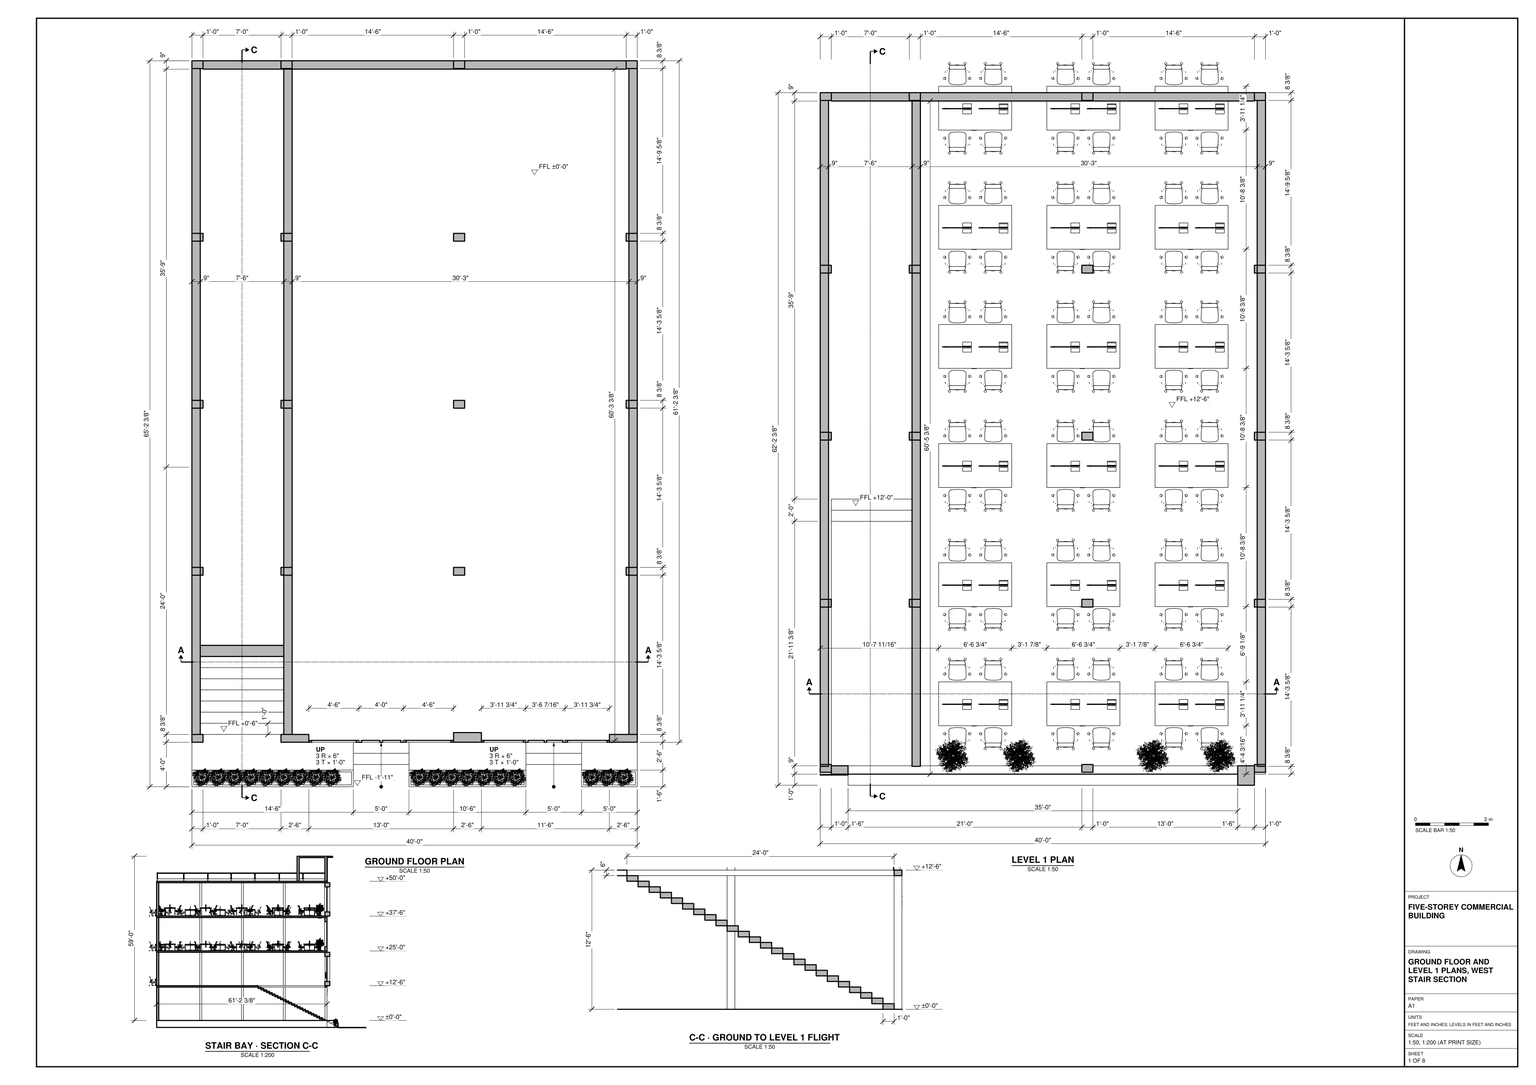
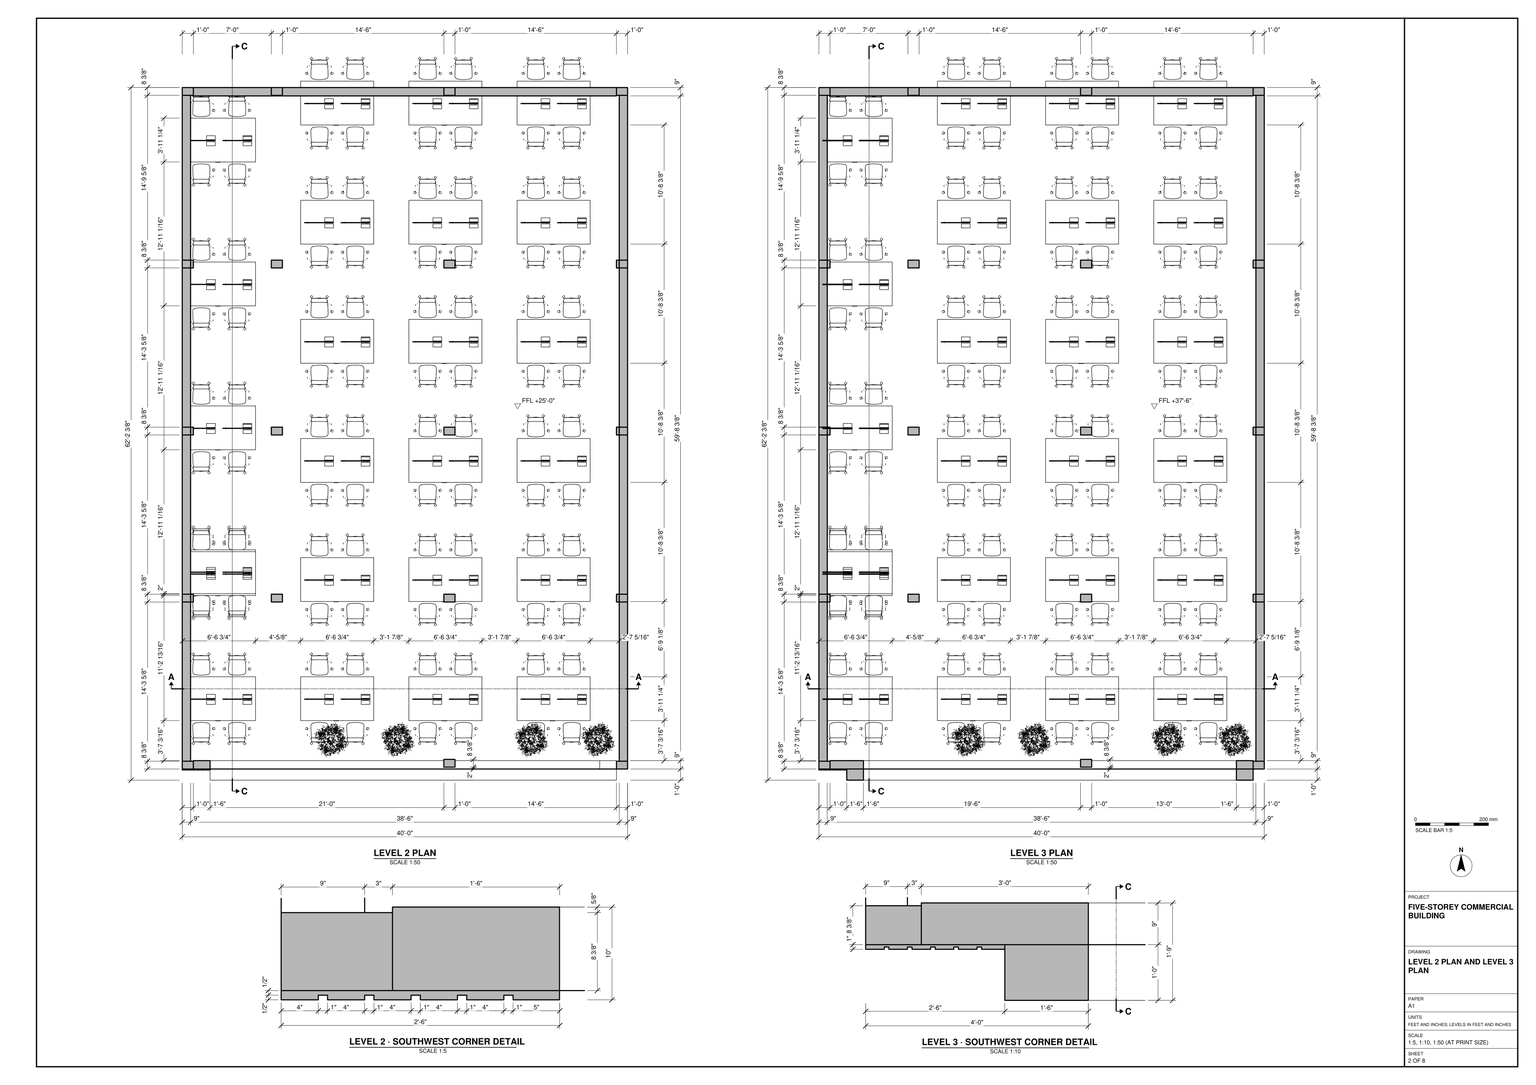
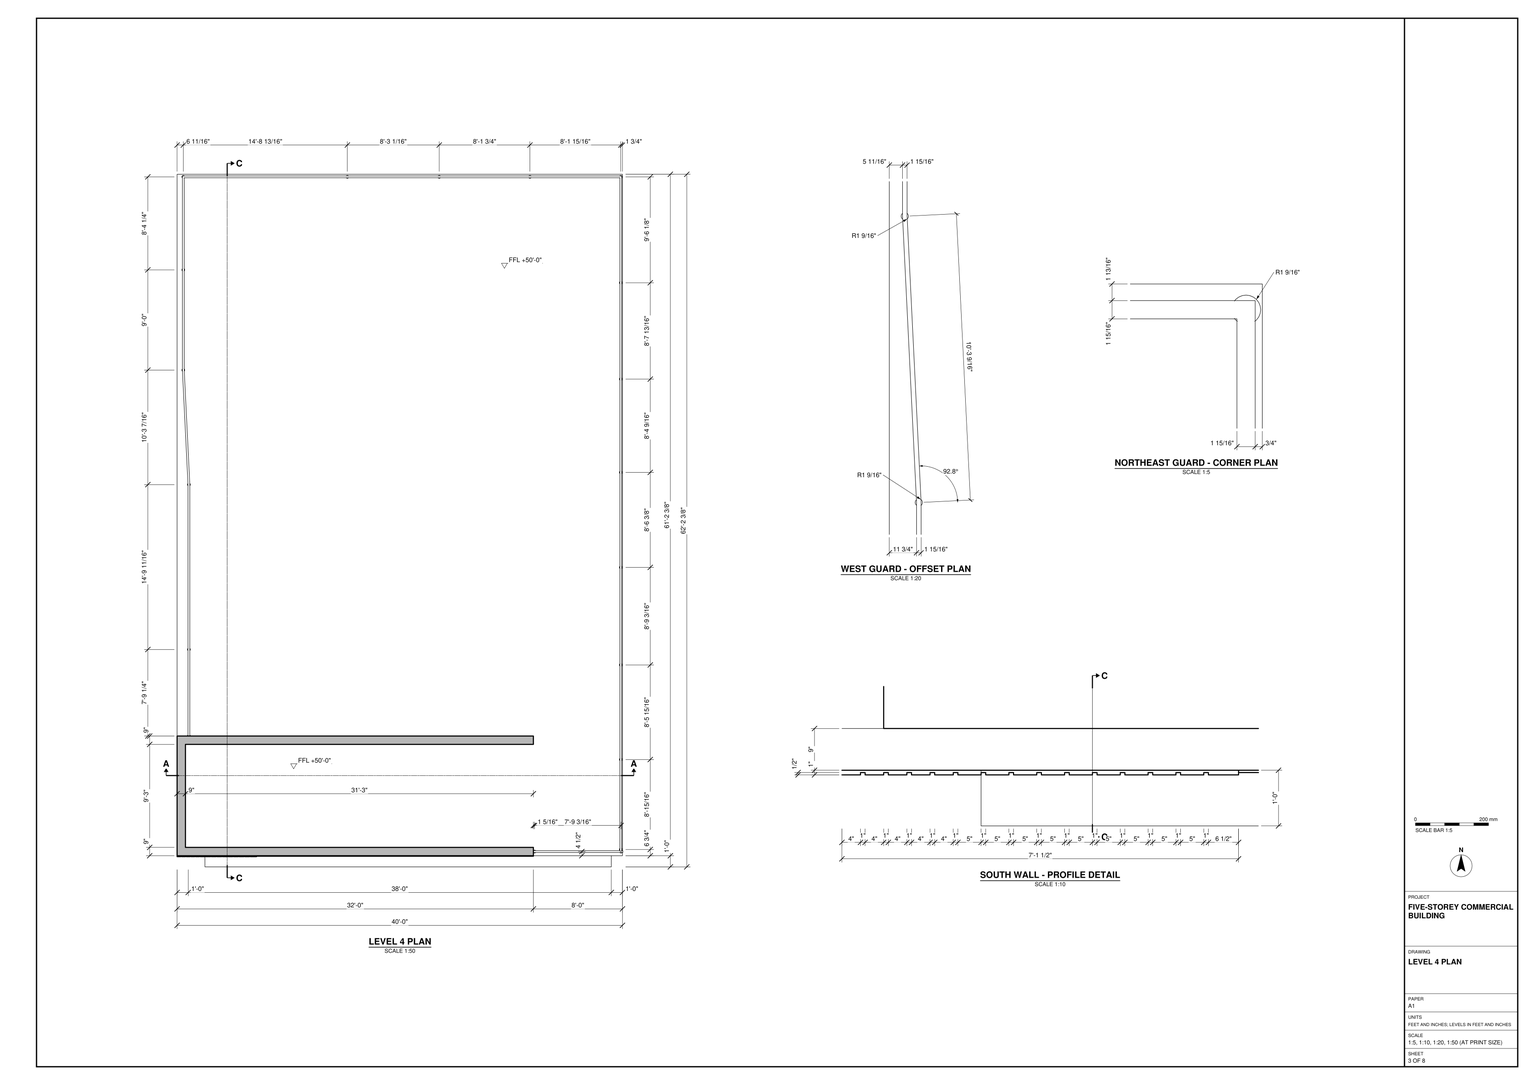
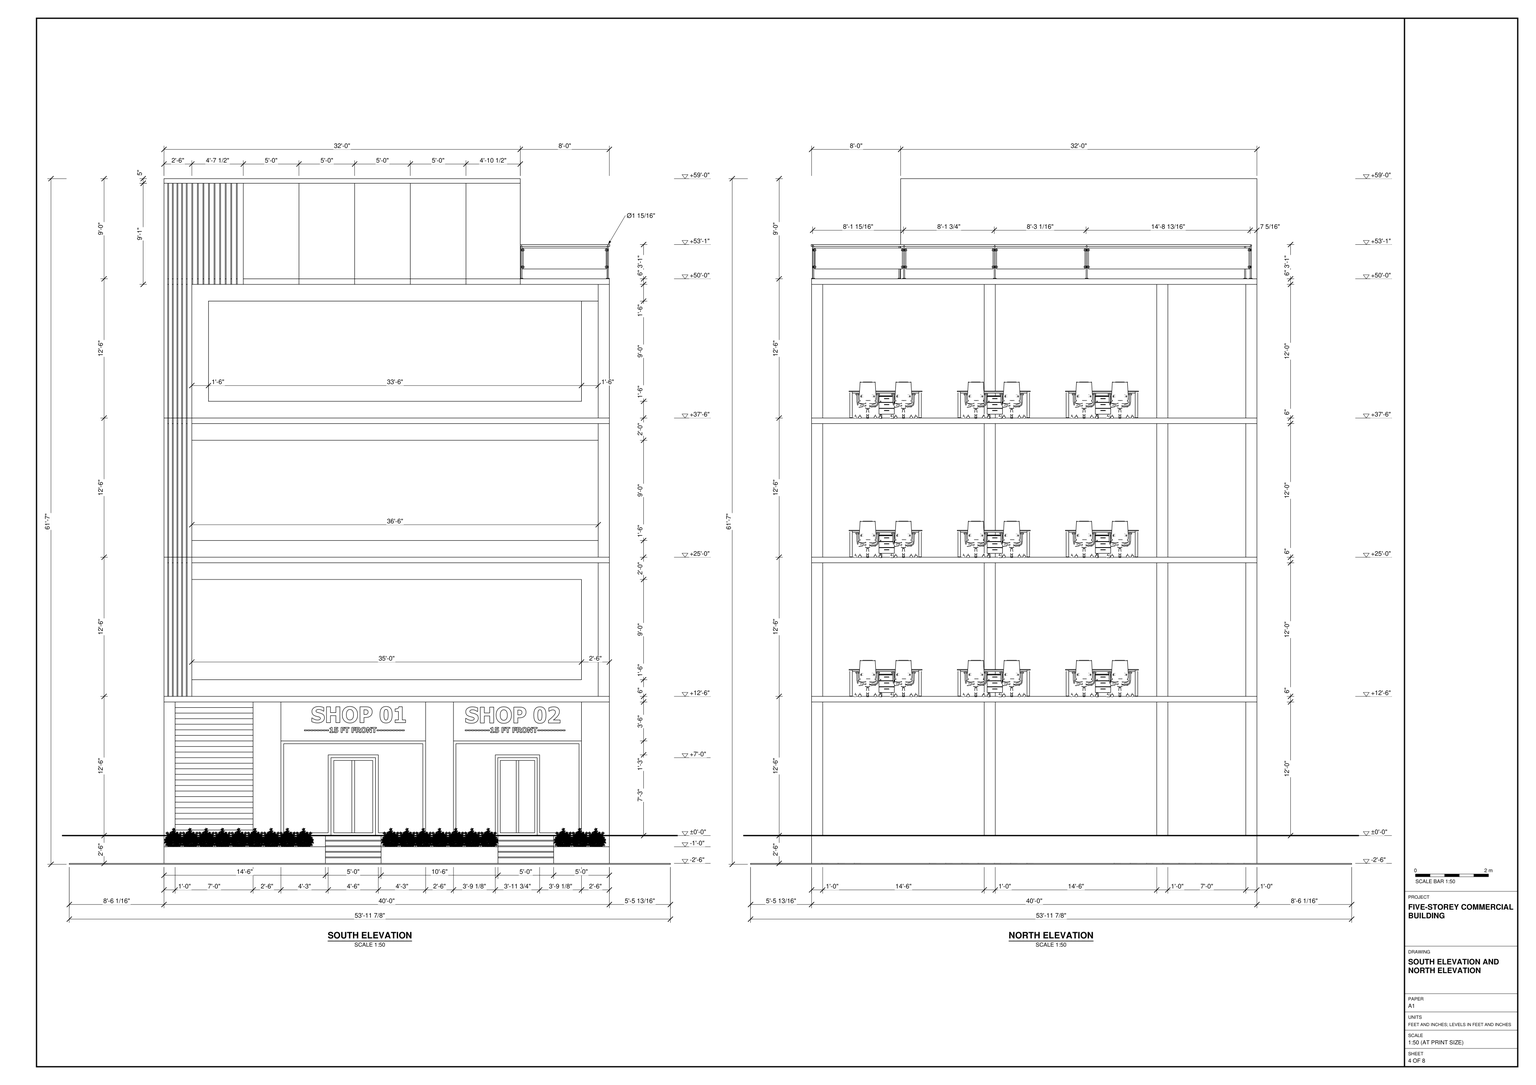
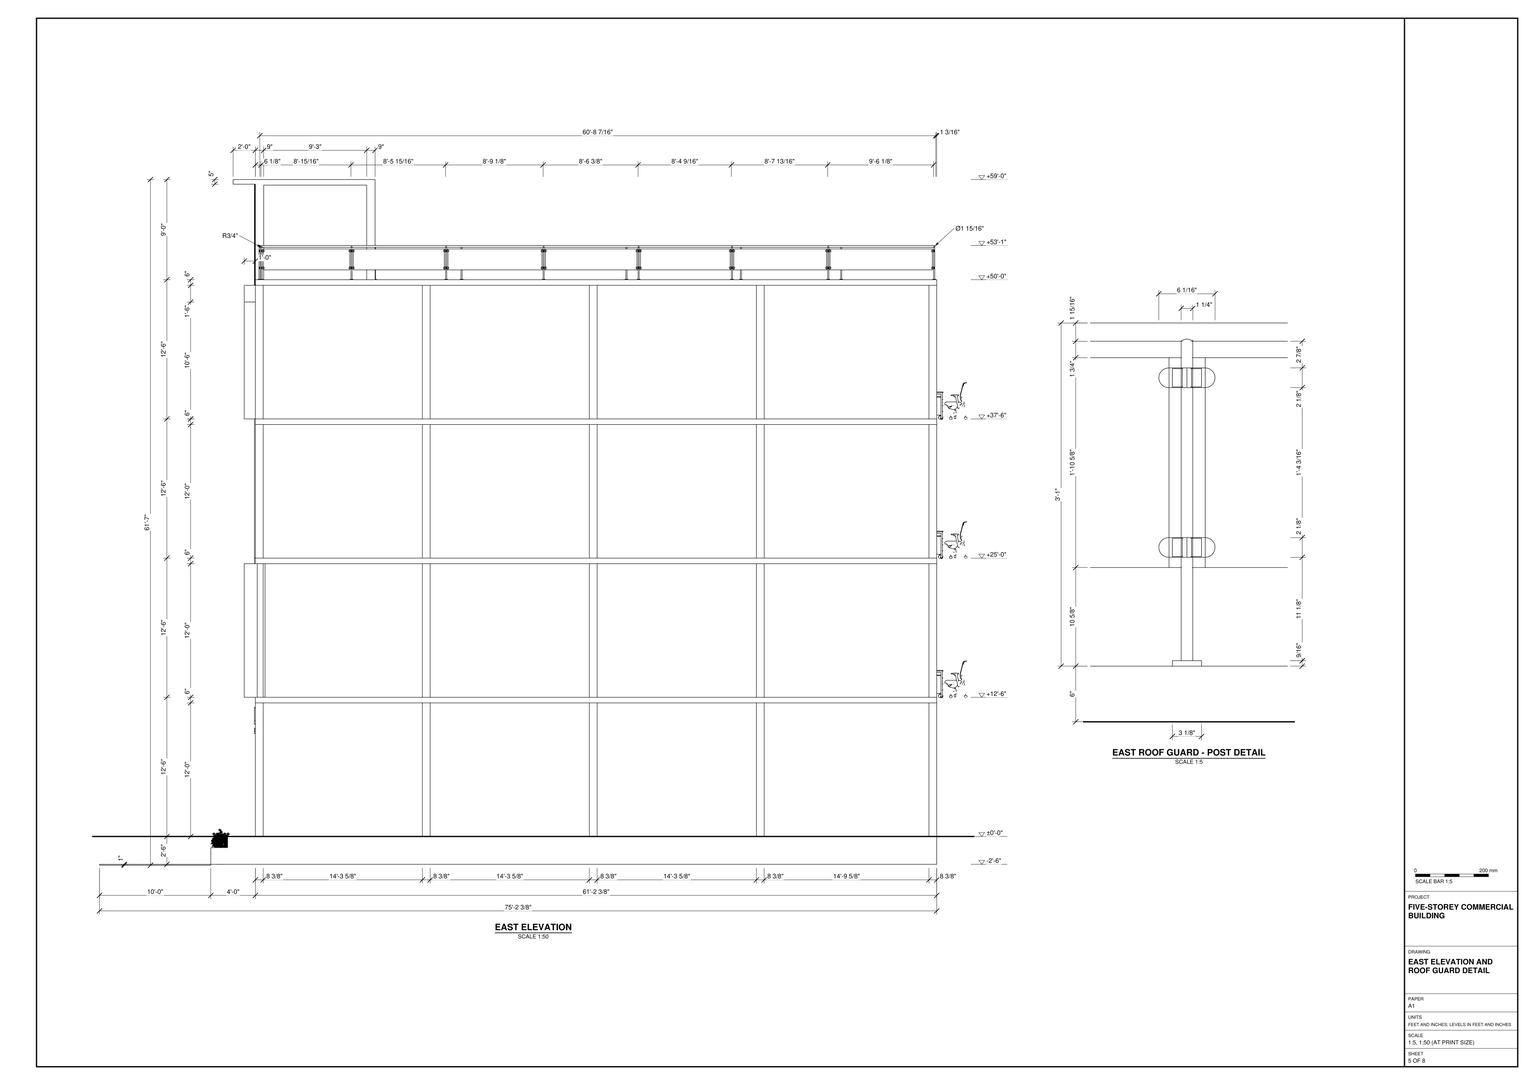
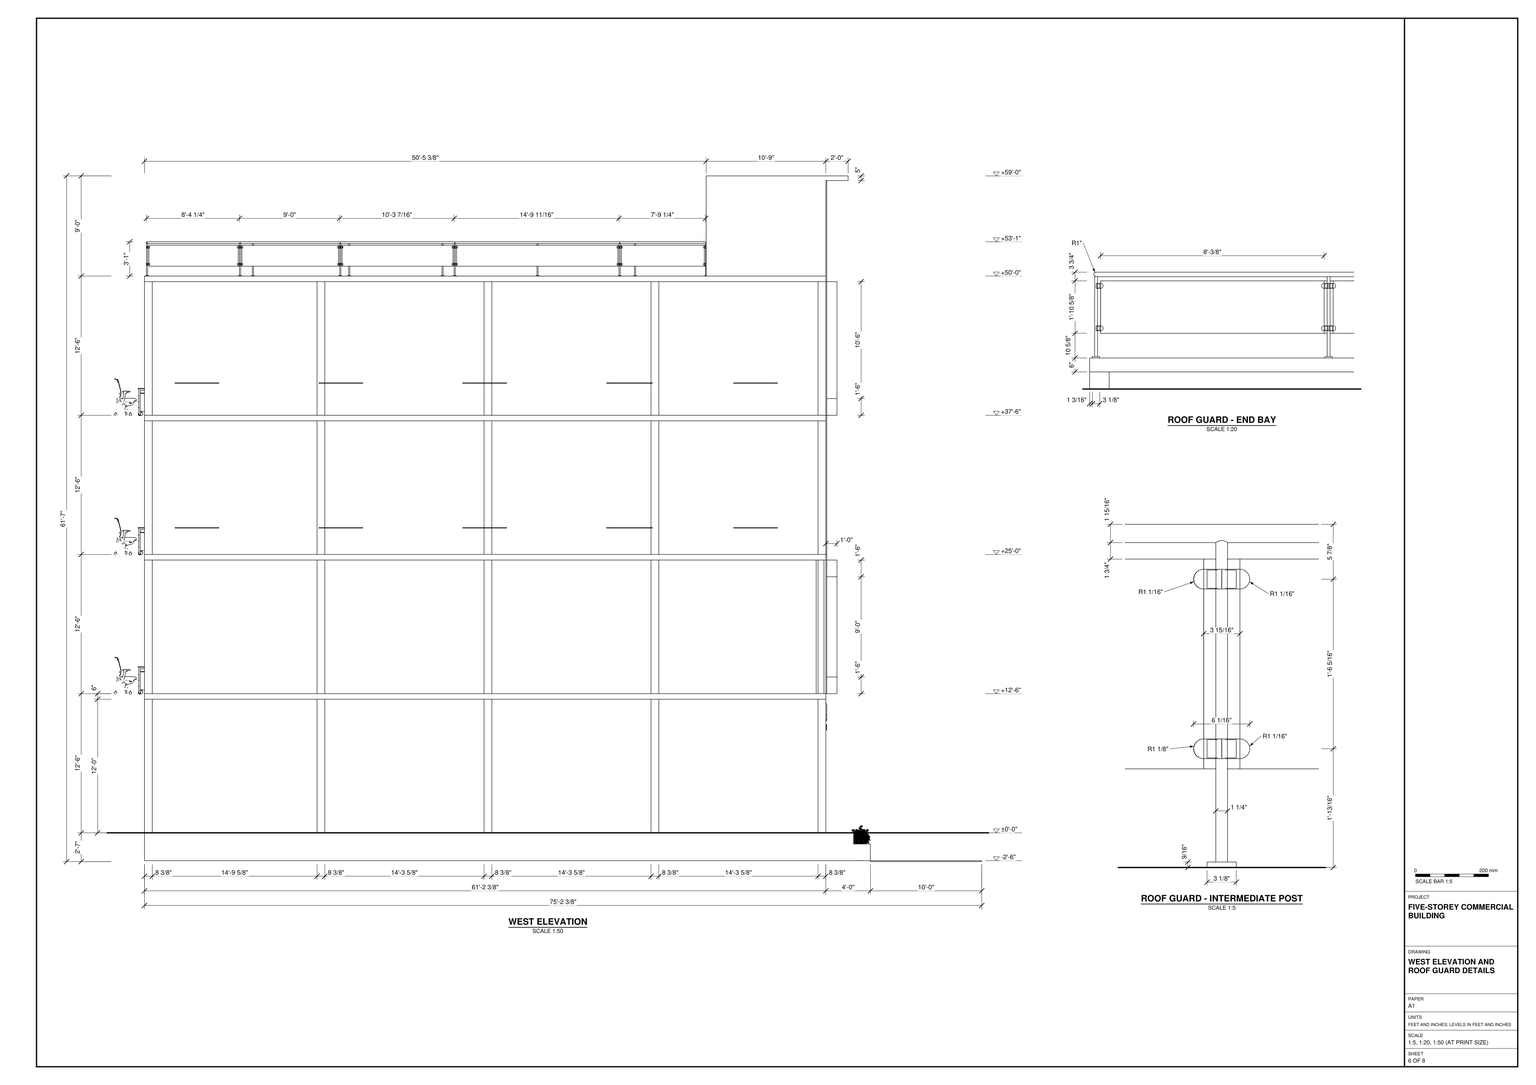
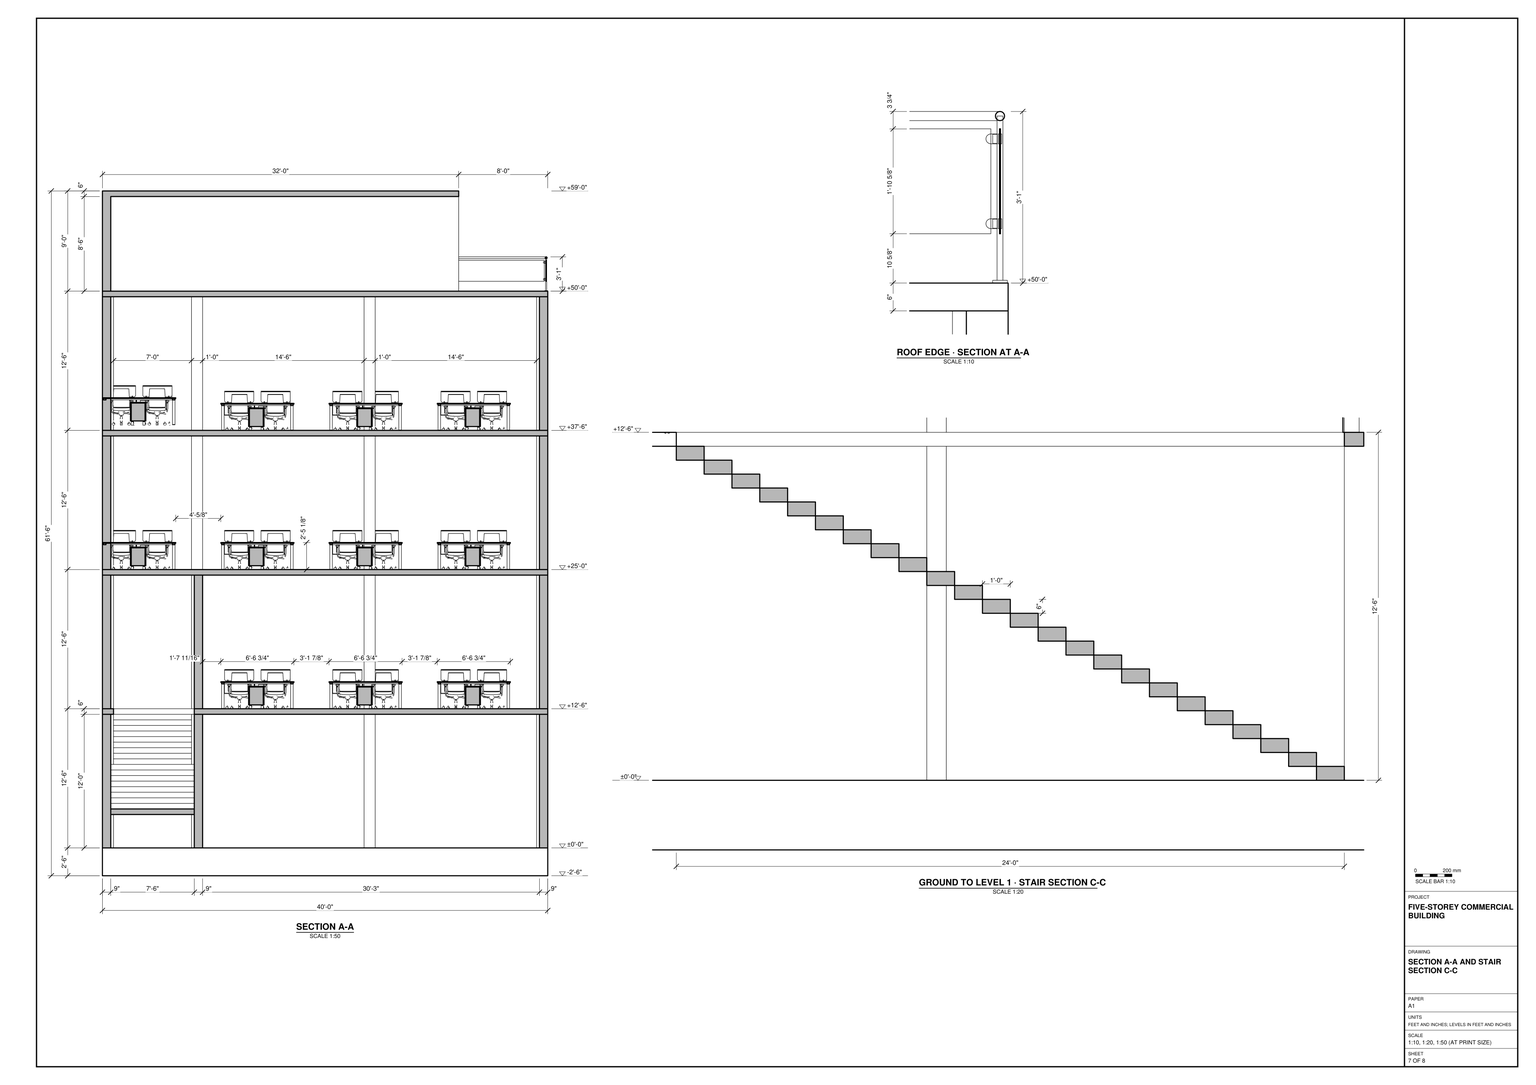
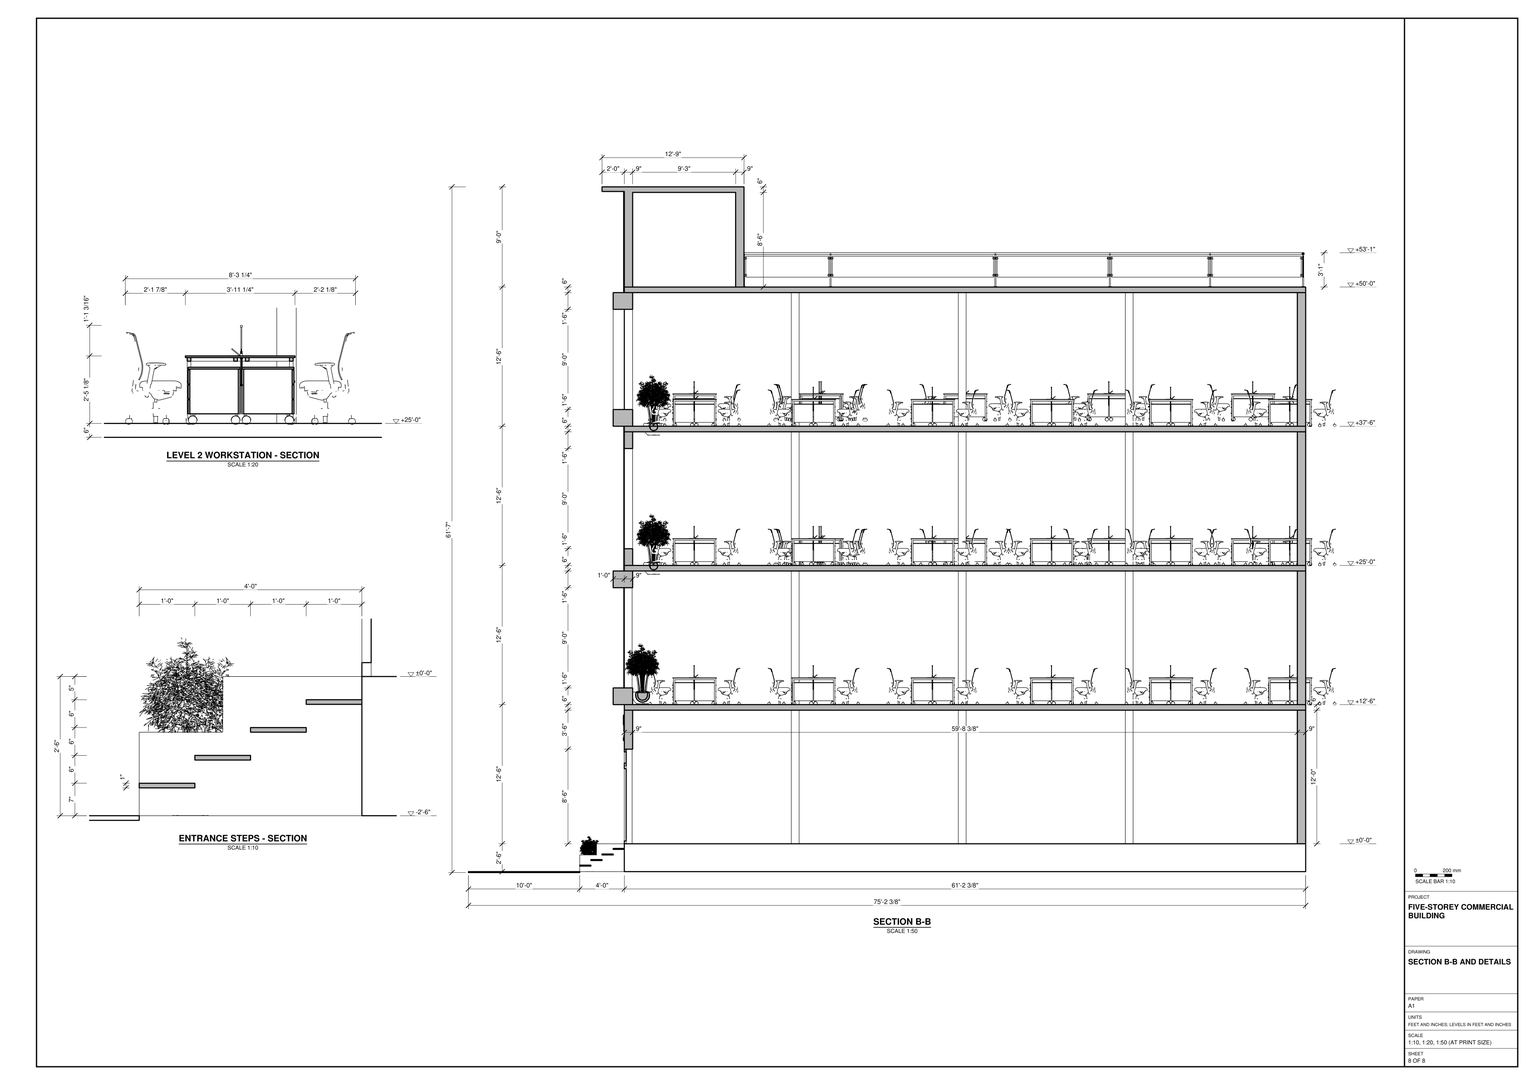
Build the five-storey commercial building in SketchUp using task_files/diagram_01.pdf. Work in feet and inches. The overall model extents are 53'-11 7/8" along X, 77'-11 3/16" along Y and 61'-7" along Z. Use the ground floor at ±0'-0" as the datum. Set Levels 1 through 4 at +12'-6", +25'-0", +37'-6" and +50'-0", respectively.

Set out the 40'-0" building width first. Follow the plans for the columns, wall thicknesses, openings and floor slabs, and the details for the projecting slab edges and corners. Keep the main ground-floor space open beside the narrow west stair bay. Model the straight flight to Level 1 and the two short flights at the south entrances. On Level 1, lay out the office tables and chairs east of the stair bay; on Levels 2 and 3, extend the workstation layout into the west bay. Match the table footprints, aisles and seating positions shown in plan.

Model the roof deck at Level 4 with its taller south-end walls and perimeter guard, including the offset along the west edge. Decor and loose items, including the plants, may be any suitable library components placed as shown. Keep shell elements such as walls, slabs and roof, and each furniture or joinery piece, in separate groups or components; use components for repeated parts. Save one SketchUp model as output_files/five_storey_commercial_building_with_a_west_stair_bay.skp.

# SketchUp Ruby script. Lengths in inches.
U = 1.inch
M = Sketchup.active_model
def pt(a) = Geom::Point3d.new(a.map { |v| v * U })
def face(e, loops, mat)
  f = e.add_face(loops[0].map { |a| pt(a) })
  loops[1..].each { |l| e.add_face(l.map { |a| pt(a) }).erase! }
  f.material = f.back_material = mat if mat
  f
end
# faces: each face lists its corners as indices into pts; further lists are holes
def faces(e, pts, list, mat = nil) = list.each { |f| face(e, (f[0].is_a?(Array) ? f : [f]).map { |l| l.map { |i| pts[i] } }, mat) }
# xy, xz, yz: faces in a plane at the given z, y or x. An outline is a flat list of corners, or four numbers for a rectangle; further outlines are holes
def ring(l) = l.size == 4 ? [[l[0], l[1]], [l[2], l[1]], [l[2], l[3]], [l[0], l[3]]] : l.each_slice(2).to_a
def flat(e, list, mat, &to3) = list.each { |f| face(e, (f[0].is_a?(Array) ? f : [f]).map { |l| ring(l).map { |u, v| to3.(u, v) } }, mat) }
def xy(e, z, list, mat = nil) = flat(e, list, mat) { |x, y| [x, y, z] }
def xz(e, y, list, mat = nil) = flat(e, list, mat) { |x, z| [x, y, z] }
def yz(e, x, list, mat = nil) = flat(e, list, mat) { |y, z| [x, y, z] }
def lines(e, pts, list) = list.each { |a, b| e.add_line(pt(pts[a]), pt(pts[b])) }
# prism: a flat outline (further loops are holes) pulled along v
def prism(e, loops, v, mat = nil)
  f = face(e, loops, mat); d = Geom::Vector3d.new(v.map { |x| x * U })
  f.pushpull(f.normal.samedirection?(d) ? d.length : -d.length)
end
def box(e, o, s, mat = nil) = prism(e, [[o, [o[0] + s[0], o[1], o[2]], [o[0] + s[0], o[1] + s[1], o[2]], [o[0], o[1] + s[1], o[2]]]], [0, 0, s[2]], mat)
def at(x, y, z, deg = 0) = Geom::Transformation.translation(pt([x, y, z])) * Geom::Transformation.rotation(ORIGIN, Z_AXIS, deg.degrees)
def axes(o, x, y, z) = Geom::Transformation.new([*x, 0, *y, 0, *z, 0, *pt(o).to_a, 1])
def part(name) = M.definitions.add(name)
# library, detail: a bought-in or finely detailed component or shape, given as its bounding box
def library(name, o, s) = part(name).tap { |d| box(d.entities, o, s) }
def detail(e, o, s) = box(e.add_group.entities, o, s)
def put(e, d, t, mat = nil) = e.add_instance(d, t).tap { |i| i.material = mat if mat }
def group(e, t, mat = nil) = e.add_group.tap { |g| g.transformation = t; g.material = mat if mat }.entities
root = M.entities
M.materials.add("[Color C07]").color = [84, 41, 0]
M.materials.add("[Color M07]").color = [58, 58, 58]
M.materials.add("[Granite Dark Gray]").color = [69, 68, 68]
M.materials.add("[Stone Vein Gray]").color = [166, 165, 165]
M.materials.add("[Translucent Glass Gray]").color = [128, 128, 128]
M.materials["[Translucent Glass Gray]"].alpha = 0.1
M.materials.add("[Translucent Glass Gray]1").color = [128, 128, 128]
M.materials["[Translucent Glass Gray]1"].alpha = 0.5
M.materials.add("[Wood Cherry Original]").color = [152, 86, 42]
c1 = library("SHOP 01",[0.84,0,0],[101.09,17.83,1])
c2 = library("SHOP 02",[0.84,0,0],[101.85,17.83,1])
c3 = library("--------15 FT FR",[0.42,0,0],[107.78,5.94,1])
c4 = part("Group\#2")
box(c4.entities,[0,0,0],[12,8.4,144])
c5 = part("Group\#43")
box(c5.entities,[0,0,0],[12,8.4,144])
c6 = part("Group\#15")
put(c6.entities,c5,at(282,0,0))
put(c6.entities,c5,at(96,0,0))
put(c6.entities,c5,at(468,0,0))
put(c6.entities,c4,at(0,0,0))
c7 = part("Group\#7")
box(c7.entities,[363,0,0],[9,717.6,144])
c8 = part("Group\#6")
box(c8.entities,[0,0,0],[9,717.6,144])
c9 = part("Group\#8")
box(c9.entities,[0,0,0],[456,9,144])
c10 = part("Group\#9")
box(c10.entities,[0,0,0],[90,12,6])
c11 = part("Group\#5")
box(c11.entities,[0,0,0],[480,734.4,6])
c12 = part("Group\#25")
xy(c12.entities,0,[[0,0,4,1],[5,0,9,1],[10,0,14,1],[15,0,19,1],[20,0,24,1],
  [25,0,30,1],[4,0.5,5,1],[9,0.5,10,1],[14,0.5,15,1],[19,0.5,20,1],
  [24,0.5,25,1]],"[Wood Cherry Original]")
xy(c12.entities,150,[[0,0,4,1],[5,0,9,1],[10,0,14,1],[15,0,19,1],[20,0,24,1],
  [25,0,30,1],[4,0.5,5,1],[9,0.5,10,1],[14,0.5,15,1],[19,0.5,20,1],
  [24,0.5,25,1]],"[Wood Cherry Original]")
xz(c12.entities,0,[[0,0,4,150],[5,0,9,150],[10,0,14,150],[15,0,19,150],[20,0,24,150],
  [25,0,30,150]],"[Wood Cherry Original]")
xz(c12.entities,0.5,[[4,0,5,150],[9,0,10,150],[14,0,15,150],[19,0,20,150],[24,0,25,150]],"[Wood Cherry Original]")
yz(c12.entities,0,[[0,0,1,150]],"[Wood Cherry Original]")
yz(c12.entities,4,[[0,0,0.5,150]],"[Wood Cherry Original]")
yz(c12.entities,5,[[0,0,0.5,150]],"[Wood Cherry Original]")
yz(c12.entities,9,[[0,0,0.5,150]],"[Wood Cherry Original]")
yz(c12.entities,10,[[0,0,0.5,150]],"[Wood Cherry Original]")
yz(c12.entities,14,[[0,0,0.5,150]],"[Wood Cherry Original]")
yz(c12.entities,15,[[0,0,0.5,150]],"[Wood Cherry Original]")
yz(c12.entities,19,[[0,0,0.5,150]],"[Wood Cherry Original]")
yz(c12.entities,20,[[0,0,0.5,150]],"[Wood Cherry Original]")
yz(c12.entities,24,[[0,0,0.5,150]],"[Wood Cherry Original]")
yz(c12.entities,25,[[0,0,0.5,150]],"[Wood Cherry Original]")
yz(c12.entities,30,[[0,0,1,150]],"[Wood Cherry Original]")
c13 = part("Group\#13")
xz(c13.entities,0,[[0,0,438,108]])
c14 = part("Group\#4")
put(c14.entities,c5,at(282,2,0))
put(c14.entities,c5,at(468,0,0))
put(c14.entities,c4,at(0,0,0))
c15 = library("Group\#27",[0,0,0],[97.125,3.15,36.98])
c16 = library("Group\#51",[0,0,0],[126.13,128.05,224.37])
c17 = library("Group\#38",[0,0,0],[126.13,128.05,224.37])
c18 = part("Group\#50")
put(c18.entities,c16,axes([288,0,0],[0.29,0,0],[0,0.29,0],[0,0,0.29]))
put(c18.entities,c16,axes([216,0,0],[0.29,0,0],[0,0.29,0],[0,0,0.29]))
put(c18.entities,c16,axes([72,0,0],[0.29,0,0],[0,0.29,0],[0,0,0.29]))
put(c18.entities,c16,axes([0,0,0],[0.29,0,0],[0,0.29,0],[0,0,0.29]))
c19 = part("Group\#44")
box(c19.entities,[0,0,0],[60,12,6])
c20 = part("Group\#48")
box(c20.entities,[0,0,0],[60,12,1])
c21 = part("Group\#49")
xy(c21.entities,0,[[0,0,54,2],[54,0,102,2],[102,0,156,2]])
xy(c21.entities,3,[[3,0,51,2],[105,0,153,2]])
xy(c21.entities,3,[[57,0,76.5,2],[79.5,0,99,2]],"[Color M07]")
xy(c21.entities,81,[[57,0,76.5,2],[79.5,0,99,2]])
xy(c21.entities,87,[[51,0,105,2]])
xy(c21.entities,99,[[3,0,153,2]])
xy(c21.entities,102,[[0,0,156,2]])
xz(c21.entities,0,[[[0,0,54,0,54,84,102,84,102,0,156,0,156,102,0,102],[3,3,3,99,153,99,153,3,105,3,105,87,51,87,51,3]],[[54,0,102,84],[57,3,99,81]],[76.5,3,79.5,81]],"[Color M07]")
xz(c21.entities,2,[[[0,0,0,102,156,102,156,0,102,0,102,84,54,84,54,0],[3,3,51,3,51,87,105,87,105,3,153,3,153,99,3,99]]])
xz(c21.entities,2,[[3,3,51,3,51,87,105,87,105,3,153,3,153,99,3,99],[57,3,76.5,81],[79.5,3,99,81]],"[Translucent Glass Gray]1")
yz(c21.entities,0,[[0,0,2,102]])
yz(c21.entities,3,[[0,3,2,99]])
yz(c21.entities,51,[[0,3,2,87]])
yz(c21.entities,57,[[0,3,2,81]],"[Color M07]")
yz(c21.entities,76.5,[[0,3,2,81]])
yz(c21.entities,79.5,[[0,3,2,81]],"[Color M07]")
yz(c21.entities,99,[[0,3,2,81]])
yz(c21.entities,105,[[0,3,2,87]])
yz(c21.entities,153,[[0,3,2,99]])
yz(c21.entities,156,[[0,0,2,102]])
p = [[54,2,84],[54,0,84],[102,2,84],[102,0,84]]
lines(c21.entities,p,[[0,1],[2,3]])
c22 = library("Group\#53",[0,0,0],[161.58,21.91,38.39])
c23 = library("Group\#54",[0,0,0],[126.58,21.91,38.39])
c24 = library("Group\#52",[0,0,0],[56.58,21.91,38.39])
c25 = library("Office+Table",[0,-0.42,0],[78.74,100.08,42.77])
c26 = part("Group\#72")
put(c26.entities,c25,at(0,0,0))
put(c26.entities,c25,at(116.625,0,0))
put(c26.entities,c25,at(233.25,0,0))
c27 = part("Group\#73")
put(c27.entities,c25,at(0,136.8125,0))
put(c27.entities,c25,at(0,134.8125,0))
put(c27.entities,c25,at(0,446.9375,0))
put(c27.entities,c25,at(0,291.875,0))
put(c27.entities,c25,at(0,602,0))
put(c27.entities,c25,at(0,0,0))
c28 = library("Group\#74",[0,0,0],[474.71,728.42,36.98])
put(root,c1,axes([260.53,168,121.34],[1,0,0],[0,0,1],[0,-1,0]))
put(root,c2,axes([426.34,168,120.97],[1,0,0],[0,0,1],[0,-1,0]))
put(root,c3,axes([252.9375,168,110.8],[1,0,0],[0,0,1],[0,-1,0]))
put(root,c3,axes([426.25,168,110.8],[1,0,0],[0,0,1],[0,-1,0]))
g1 = group(root,at(102.0625,168,0))
xy(g1,-30,[[0,-48,0,734.4,480,734.4,480,-48,420,-48,420,0,360,0,360,-48,234,-48,234,0,174,0,174,-48]])
xy(g1,-24,[[2,-46,172,-32],[236,-46,358,-32],[422,-46,478,-32]])
xy(g1,-12,[[[0,-48,174,-30],[2,-46,172,-32]],[[234,-48,360,-30],[236,-46,358,-32]],[[420,-48,480,-30],[422,-46,478,-32]]])
xy(g1,0,[[0,-30,174,-30,174,0,420,0,420,-30,480,-30,480,734.4,0,734.4],[234,-30,360,0]])
xz(g1,-48,[[0,-30,174,-12],[234,-30,360,-12],[420,-30,480,-12]])
xz(g1,-46,[[2,-24,172,-12],[236,-24,358,-12],[422,-24,478,-12]])
xz(g1,-32,[[2,-24,172,-12],[236,-24,358,-12],[422,-24,478,-12]])
xz(g1,-30,[[0,-12,174,0],[234,-12,360,0],[420,-12,480,0]])
xz(g1,0,[[174,-30,234,0],[360,-30,420,0]])
xz(g1,734.4,[[0,-30,480,0]])
yz(g1,0,[[-48,-30,-48,-12,-30,-12,-30,0,734.4,0,734.4,-30]])
yz(g1,2,[[-46,-24,-32,-12]])
yz(g1,172,[[-46,-24,-32,-12]])
yz(g1,174,[[-48,-30,0,-30,0,0,-30,0,-30,-12,-48,-12]])
yz(g1,234,[[-48,-30,-48,-12,-30,-12,-30,0,0,0,0,-30]])
yz(g1,236,[[-46,-24,-32,-12]])
yz(g1,358,[[-46,-24,-32,-12]])
yz(g1,360,[[-48,-30,0,-30,0,0,-30,0,-30,-12,-48,-12]])
yz(g1,420,[[-48,-30,-48,-12,-30,-12,-30,0,0,0,0,-30]])
yz(g1,422,[[-46,-24,-32,-12]])
yz(g1,478,[[-46,-24,-32,-12]])
yz(g1,480,[[-48,-30,734.4,-30,734.4,0,-30,0,-30,-12,-48,-12]])
g2 = group(root,at(102.0625,168,0))
g3 = group(g2,at(282,2,0))
box(g3,[0,-2,0],[30,10.4,144])
g4 = group(g2,at(96,0,0))
box(g4,[0,0,0],[30,8.4,144])
g5 = group(g2,at(468,0,0))
box(g5,[-18,0,0],[30,8.4,144])
put(g2,c4,at(0,0,0))
put(root,c6,at(102.0625,348,0))
put(root,c6,at(102.0625,528,0))
put(root,c6,at(102.0625,708,0))
put(root,c6,at(102.0625,894,0))
g6 = group(root,at(102.0625,168,144))
prism(g6,[[[480,734.4,0],[480,0,0],[0,0,0],[0,734.4,0]],[[12,8.4,0],[99,8.4,0],[99,296.4,0],[12,296.4,0]]],[0,0,6])
put(root,c7,at(210.0625,176.4,0))
put(root,c8,at(102.0625,176.4,0))
put(root,c9,at(114.0625,893.4,0))
put(root,c8,at(201.0625,176.4,0))
g7 = group(root,at(111.0625,176.4,0))
put(g7,c10,at(0,12,6),"[Stone Vein Gray]")
put(g7,c10,at(0,0,0),"[Stone Vein Gray]")
put(g7,c10,at(0,24,12),"[Stone Vein Gray]")
put(g7,c10,at(0,36,18),"[Stone Vein Gray]")
put(g7,c10,at(0,48,24),"[Stone Vein Gray]")
put(g7,c10,at(0,60,30),"[Stone Vein Gray]")
put(g7,c10,at(0,72,36),"[Stone Vein Gray]")
put(g7,c10,at(0,84,42),"[Stone Vein Gray]")
put(g7,c10,at(0,96,48),"[Stone Vein Gray]")
put(g7,c10,at(0,108,54),"[Stone Vein Gray]")
put(g7,c10,at(0,120,60),"[Stone Vein Gray]")
put(g7,c10,at(0,132,66),"[Stone Vein Gray]")
put(g7,c10,at(0,144,72),"[Stone Vein Gray]")
put(g7,c10,at(0,156,78),"[Stone Vein Gray]")
put(g7,c10,at(0,168,84),"[Stone Vein Gray]")
put(g7,c10,at(0,180,90),"[Stone Vein Gray]")
put(g7,c10,at(0,192,96),"[Stone Vein Gray]")
put(g7,c10,at(0,204,102),"[Stone Vein Gray]")
put(g7,c10,at(0,216,108),"[Stone Vein Gray]")
put(g7,c10,at(0,228,114))
put(g7,c10,at(0,240,120),"[Stone Vein Gray]")
put(g7,c10,at(0,252,126),"[Stone Vein Gray]")
put(g7,c10,at(0,264,132),"[Stone Vein Gray]")
put(g7,c10,at(0,276,138),"[Stone Vein Gray]")
g8 = group(root,at(102.0625,167,150))
put(g8,c11,at(0,1,144))
put(g8,c12,at(0,0,0))
put(g8,c6,at(0,361,0))
put(g8,c6,at(0,181,0))
g9 = group(g8,at(0,3,0))
put(g9,c5,at(282,0,0))
put(g9,c5,at(468,0,0))
put(g9,c4,at(0,0,0))
put(g8,c6,at(0,541,0))
put(g8,c7,at(108,9.4,0))
put(g8,c6,at(0,727,0))
put(g8,c9,at(12,726.4,0))
put(g8,c8,at(99,9.4,0))
put(g8,c8,at(0,9.4,0))
g10 = group(g8,at(12,1,0))
xy(g10,0,[[18,-12,18,0,0,0,0,9,456,9,456,-12]])
xy(g10,18,[[18,-12,438,9]])
xy(g10,126,[[18,-12,438,9]])
xy(g10,144,[[18,-12,456,-12,456,9,0,9,0,0,18,0]])
xz(g10,-12,[[18,0,456,0,456,144,18,144,18,126,438,126,438,18,18,18]])
xz(g10,0,[[0,0,18,144]])
xz(g10,9,[[[0,0,456,144],[18,18,438,126]]])
yz(g10,0,[[0,0,9,144]])
yz(g10,18,[[-12,0,0,18],[0,18,9,126],[-12,126,0,144]])
yz(g10,438,[[-12,18,9,126]])
yz(g10,456,[[-12,0,9,144]])
g11 = group(g10,at(18,0,18),"[Translucent Glass Gray]")
xz(g11,0,[[0,0,420,108]])
g12 = group(root,at(102.0625,167,300))
put(g12,c6,at(0,541,0))
put(g12,c7,at(108,9.4,0))
put(g12,c12,at(0,0,0))
g13 = group(g12,at(12,1,0))
xy(g13,0,[[0,0,456,9]])
xy(g13,18,[[18,0,438,9],[438,0,456,9]])
xy(g13,126,[[18,0,438,9],[438,0,456,9]])
xy(g13,144,[[0,0,456,9]])
xz(g13,0,[[0,0,18,144],[18,0,456,18],[18,126,456,144]])
xz(g13,9,[[0,0,0,144,456,144,456,126,18,126,18,18,456,18,456,0]])
yz(g13,0,[[0,0,9,144]])
yz(g13,18,[[0,18,9,126]])
yz(g13,456,[[0,0,9,18],[0,126,9,144]])
p = [[456,9,18],[456,9,126]]
lines(g13,p,[[0,1]])
put(g13,c13,at(18,0,18),"[Translucent Glass Gray]")
put(g12,c6,at(0,181,0))
put(g12,c6,at(0,361,0))
put(g12,c8,at(0,9.4,0))
put(g12,c9,at(12,726.4,0))
put(g12,c11,at(0,1,144))
put(g12,c14,at(0,1,0))
put(g12,c6,at(0,727,0))
g14 = group(root,at(102.0625,167,450))
put(g14,c6,at(0,541,0))
put(g14,c7,at(108,9.4,0))
g15 = group(g14,at(12,1,0))
xy(g15,0,[[18,-12,18,0,0,0,0,9,456,9,456,-12]])
xy(g15,18,[[36,-12,438,9]])
xy(g15,126,[[36,-12,438,9],[438,-12,456,9]])
xy(g15,144,[[18,-12,456,-12,456,9,0,9,0,0,18,0]])
xz(g15,-12,[[18,0,456,0,456,126,438,126,438,18,36,18,36,126,456,126,456,144,18,144]])
xz(g15,0,[[0,0,18,144]])
xz(g15,9,[[0,0,0,144,456,144,456,126,36,126,36,18,438,18,438,126,456,126,456,0]])
yz(g15,0,[[0,0,9,144]])
yz(g15,18,[[-12,0,0,18],[-12,18,0,144]])
yz(g15,36,[[-12,18,0,126],[0,18,9,126]])
yz(g15,438,[[-12,18,9,126]])
yz(g15,456,[[-12,0,9,126],[-12,126,9,144]])
put(g15,c13,at(18,0,18),"[Translucent Glass Gray]")
put(g14,c6,at(0,181,0))
put(g14,c6,at(0,361,0))
put(g14,c8,at(0,9.4,0))
put(g14,c9,at(12,726.4,0))
put(g14,c11,at(0,1,144))
put(g14,c14,at(0,1,0))
put(g14,c6,at(0,727,0))
g16 = group(g14,at(0,0,0))
xy(g16,0,[[0,0,4,1],[5,0,9,1],[10,0,14,1],[15,0,19,1],[20,0,24,1],
  [25,0,30,1],[4,0.5,5,1],[9,0.5,10,1],[14,0.5,15,1],[19,0.5,20,1],
  [24,0.5,25,1]],"[Wood Cherry Original]")
xy(g16,144,[[31,0,31,0.5,30,0.5,30,1,85.5,1,85.5,0,79,0,79,0.5,78,0.5,78,0,73,0,73,0.5,72,0.5,72,0,67,0,67,0.5,66,0.5,66,0,61,0,61,0.5,60,0.5,60,0,55,0,55,0.5,54,0.5,54,0,49,0,49,0.5,48,0.5,48,0,43,0,43,0.5,42,0.5,42,0,37,0,37,0.5,36,0.5,36,0]],"[Wood Cherry Original]")
xy(g16,253,[[0,0,4,0,4,0.5,5,0.5,5,0,9,0,9,0.5,10,0.5,10,0,14,0,14,0.5,15,0.5,15,0,19,0,19,0.5,20,0.5,20,0,24,0,24,0.5,25,0.5,25,0,30,0,30,0.5,31,0.5,31,0,36,0,36,0.5,37,0.5,37,0,42,0,42,0.5,43,0.5,43,0,48,0,48,0.5,49,0.5,49,0,54,0,54,0.5,55,0.5,55,0,60,0,60,0.5,61,0.5,61,0,66,0,66,0.5,67,0.5,67,0,72,0,72,0.5,73,0.5,73,0,78,0,78,0.5,79,0.5,79,0,85.5,0,85.5,1,0,1]],"[Wood Cherry Original]")
xz(g16,0,[[0,0,4,253],[5,0,9,253],[10,0,14,253],[15,0,19,253],[20,0,24,253],
  [25,0,30,253],[31,144,36,253],[37,144,42,253],[43,144,48,253],[49,144,54,253],
  [55,144,60,253],[61,144,66,253],[67,144,72,253],[73,144,78,253],[79,144,85.5,253]],"[Wood Cherry Original]")
xz(g16,0.5,[[4,0,5,253],[9,0,10,253],[14,0,15,253],[19,0,20,253],[24,0,25,253],
  [30,144,31,253],[36,144,37,253],[42,144,43,253],[48,144,49,253],[54,144,55,253],
  [60,144,61,253],[66,144,67,253],[72,144,73,253],[78,144,79,253]],"[Wood Cherry Original]")
xz(g16,1,[[30,144,85.5,253]],"[Wood Cherry Original]")
yz(g16,0,[[0,0,1,253]],"[Wood Cherry Original]")
yz(g16,4,[[0,0,0.5,253]],"[Wood Cherry Original]")
yz(g16,5,[[0,0,0.5,253]],"[Wood Cherry Original]")
yz(g16,9,[[0,0,0.5,253]],"[Wood Cherry Original]")
yz(g16,10,[[0,0,0.5,253]],"[Wood Cherry Original]")
yz(g16,14,[[0,0,0.5,253]],"[Wood Cherry Original]")
yz(g16,15,[[0,0,0.5,253]],"[Wood Cherry Original]")
yz(g16,19,[[0,0,0.5,253]],"[Wood Cherry Original]")
yz(g16,20,[[0,0,0.5,253]],"[Wood Cherry Original]")
yz(g16,24,[[0,0,0.5,253]],"[Wood Cherry Original]")
yz(g16,25,[[0,0,0.5,253]],"[Wood Cherry Original]")
yz(g16,30,[[0,0,1,144],[0,144,0.5,253]],"[Wood Cherry Original]")
yz(g16,31,[[0,144,0.5,253]],"[Wood Cherry Original]")
yz(g16,36,[[0,144,0.5,253]],"[Wood Cherry Original]")
yz(g16,37,[[0,144,0.5,253]],"[Wood Cherry Original]")
yz(g16,42,[[0,144,0.5,253]],"[Wood Cherry Original]")
yz(g16,43,[[0,144,0.5,253]],"[Wood Cherry Original]")
yz(g16,48,[[0,144,0.5,253]],"[Wood Cherry Original]")
yz(g16,49,[[0,144,0.5,253]],"[Wood Cherry Original]")
yz(g16,54,[[0,144,0.5,253]],"[Wood Cherry Original]")
yz(g16,55,[[0,144,0.5,253]],"[Wood Cherry Original]")
yz(g16,60,[[0,144,0.5,253]],"[Wood Cherry Original]")
yz(g16,61,[[0,144,0.5,253]],"[Wood Cherry Original]")
yz(g16,66,[[0,144,0.5,253]],"[Wood Cherry Original]")
yz(g16,67,[[0,144,0.5,253]],"[Wood Cherry Original]")
yz(g16,72,[[0,144,0.5,253]],"[Wood Cherry Original]")
yz(g16,73,[[0,144,0.5,253]],"[Wood Cherry Original]")
yz(g16,78,[[0,144,0.5,253]],"[Wood Cherry Original]")
yz(g16,79,[[0,144,0.5,253]],"[Wood Cherry Original]")
yz(g16,85.5,[[0,144,1,253]],"[Wood Cherry Original]")
p = [[30,0,253],[30,0,253.21]]
lines(g16,p,[[0,1]])
g17 = group(root,at(102.0625,168,600))
xy(g17,0,[[0,0,384,9],[0,9,9,120],[0,120,384,129]])
xy(g17,102,[[9,9,384,120]])
xy(g17,103,[[0,-24,384,0]])
xy(g17,108,[[0,-24,384,129]])
xz(g17,-24,[[0,103,384,108]])
xz(g17,0,[[0,0,384,103]])
xz(g17,9,[[9,0,384,102]])
xz(g17,120,[[9,0,384,102]])
xz(g17,129,[[0,0,384,108]])
yz(g17,0,[[0,0,0,103,-24,103,-24,108,129,108,129,0]])
yz(g17,9,[[9,0,120,102]])
yz(g17,384,[[0,0,9,0,9,102,120,102,120,0,129,0,129,108,-24,108,-24,103,0,103]])
g18 = group(root,at(187.5625,167.5,600))
xy(g18,-6,[[0,0,298.5,0.5]])
xy(g18,103,[[0,0,298.5,0.5]])
xz(g18,0,[[0,-6,60,103],[60,-6,120,103],[120,-6,180,103],[180,-6,240,103],[240,-6,298.5,103]],"[Color C07]")
xz(g18,0.5,[[0,-6,298.5,103]])
yz(g18,0,[[0,-6,0.5,103]])
yz(g18,298.5,[[0,-6,0.5,103]])
put(root,c15,at(485.39,170.93,600))
g19 = group(root,at(226.05,168.88,150.875))
put(g19,c16,axes([288,0,0],[0.29,0,0],[0,0.29,0],[0,0,0.29]))
put(g19,c16,axes([216,0,0],[0.29,0,0],[0,0.29,0],[0,0,0.29]))
put(g19,c16,axes([72,0,0],[0.29,0,0],[0,0.29,0],[0,0,0.29]))
put(g19,c17,axes([0,0,0],[0.29,0,0],[0,0.29,0],[0,0,0.29]))
put(root,c18,at(244.05,180.88,290.35))
put(root,c18,at(244.05,180.88,440.35))
g20 = group(root,at(210.0625,168,102),"[Color C07]")
xy(g20,0,[[18,0,174,9],[204,0,342,9]])
xy(g20,42,[[18,0,174,9],[174,0,204,9],[204,0,342,9]])
xz(g20,0,[[18,0,174,42],[204,0,342,42]])
xz(g20,9,[[18,0,174,42],[204,0,342,42]])
yz(g20,18,[[0,0,9,42]])
yz(g20,174,[[0,0,9,42]])
yz(g20,204,[[0,0,9,42]])
yz(g20,342,[[0,0,9,42]])
p = [[204,10.4,0],[204,9,0]]
lines(g20,p,[[0,1]])
g21 = group(root,at(462.0625,120,-30),"[Granite Dark Gray]")
put(g21,c19,at(0,24,12))
g22 = group(g21,at(0,0,0))
put(g22,c19,at(0,36,18))
g23 = group(g22,at(0,12,0))
prism(g23,[[[0,0,0],[0,0,6],[0,12,6],[0,12,12],[0,24,12],[0,24,18],[0,36,18],[0,36,0]]],[60,0,0])
put(g22,c19,at(0,12,6))
put(g22,c19,at(0,0,0))
put(root,c20,at(276.0625,156,-6),"[Stone Vein Gray]")
put(root,c20,at(276.0625,144,-12),"[Stone Vein Gray]")
put(root,c20,at(276.0625,132,-18),"[Stone Vein Gray]")
put(root,c20,at(276.0625,120,-24),"[Stone Vein Gray]")
put(root,c20,at(462.0625,156,-6),"[Stone Vein Gray]")
put(root,c20,at(462.0625,144,-12),"[Stone Vein Gray]")
put(root,c20,at(462.0625,132,-18),"[Stone Vein Gray]")
put(root,c20,at(462.0625,120,-24),"[Stone Vein Gray]")
put(root,c21,at(228.0625,168,0))
put(root,c21,axes([414.0625,168,0],[0.88462,0,0],[0,1,0],[0,0,1]))
put(root,c22,at(102.0625,120,-30))
put(root,c23,at(336.0625,120,-30))
put(root,c24,at(522.0625,120,-30))
g24 = group(root,at(0,0,-31),"[Color M07]")
box(g24,[0,0,0],[647.875,120,1])
put(root,c26,at(229.73,194.06,149.51))
g25 = group(root,at(229.73,194.06,299.51))
put(g25,c25,at(0,0,0))
put(g25,c25,at(116.625,0,0))
put(g25,c25,at(233.25,0,0))
put(g25,c27,at(-127.375,0,0))
put(g25,c27,at(-127.375,0,156))
put(root,c26,at(229.73,194.06,449.51))
put(root,c26,at(229.73,322.43,299.51))
put(root,c26,at(229.73,322.43,449.51))
put(root,c26,at(229.73,322.43,149.51))
put(root,c26,at(229.73,450.81,449.51))
put(root,c26,at(229.73,450.81,149.51))
put(root,c26,at(229.73,450.81,299.51))
put(root,c26,at(229.73,579.18,299.51))
put(root,c26,at(229.73,579.18,449.51))
put(root,c26,at(229.73,579.18,149.51))
put(root,c26,at(229.73,707.56,449.51))
put(root,c26,at(229.73,707.56,299.51))
put(root,c26,at(229.73,707.56,149.51))
put(root,c26,at(229.73,835.93,449.51))
put(root,c26,at(229.73,835.93,299.51))
put(root,c26,at(229.73,835.93,149.51))
put(root,c28,at(107.17,172.78,600))
